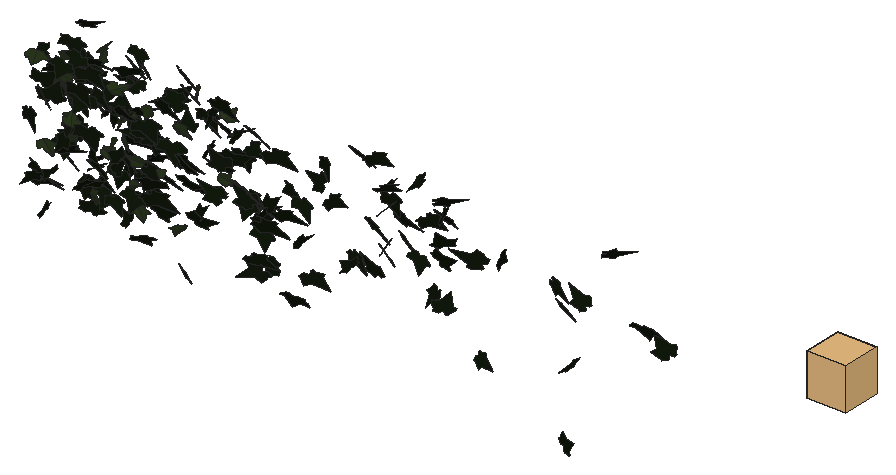
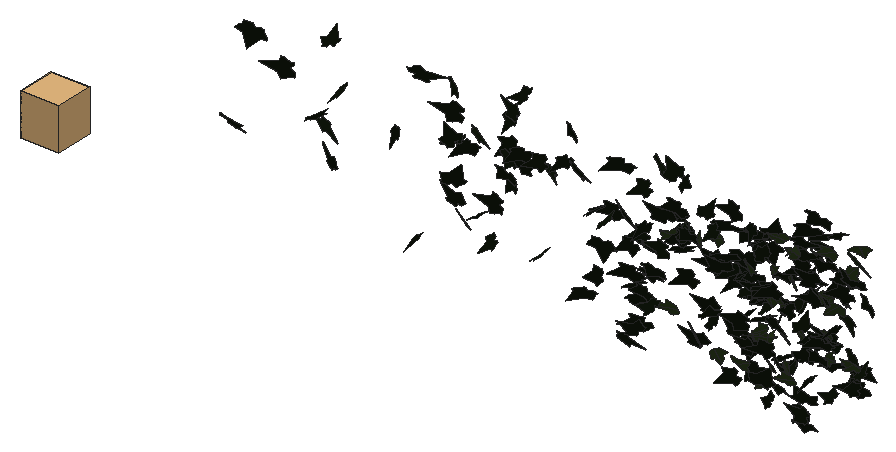
# SketchUp Ruby script. Lengths in millimetres.
U = 1.mm
M = Sketchup.active_model
def pt(a) = Geom::Point3d.new(a.map { |v| v * U })
def face(e, loops, mat)
  f = e.add_face(loops[0].map { |a| pt(a) })
  loops[1..].each { |l| e.add_face(l.map { |a| pt(a) }).erase! }
  f.material = f.back_material = mat if mat
  f
end
# faces: each face lists its corners as indices into pts; further lists are holes
def faces(e, pts, list, mat = nil) = list.each { |f| face(e, (f[0].is_a?(Array) ? f : [f]).map { |l| l.map { |i| pts[i] } }, mat) }
# xy, xz, yz: faces in a plane at the given z, y or x. An outline is a flat list of corners, or four numbers for a rectangle; further outlines are holes
def ring(l) = l.size == 4 ? [[l[0], l[1]], [l[2], l[1]], [l[2], l[3]], [l[0], l[3]]] : l.each_slice(2).to_a
def flat(e, list, mat, &to3) = list.each { |f| face(e, (f[0].is_a?(Array) ? f : [f]).map { |l| ring(l).map { |u, v| to3.(u, v) } }, mat) }
def xy(e, z, list, mat = nil) = flat(e, list, mat) { |x, y| [x, y, z] }
def xz(e, y, list, mat = nil) = flat(e, list, mat) { |x, z| [x, y, z] }
def yz(e, x, list, mat = nil) = flat(e, list, mat) { |y, z| [x, y, z] }
def lines(e, pts, list) = list.each { |a, b| e.add_line(pt(pts[a]), pt(pts[b])) }
# prism: a flat outline (further loops are holes) pulled along v
def prism(e, loops, v, mat = nil)
  f = face(e, loops, mat); d = Geom::Vector3d.new(v.map { |x| x * U })
  f.pushpull(f.normal.samedirection?(d) ? d.length : -d.length)
end
def box(e, o, s, mat = nil) = prism(e, [[o, [o[0] + s[0], o[1], o[2]], [o[0] + s[0], o[1] + s[1], o[2]], [o[0], o[1] + s[1], o[2]]]], [0, 0, s[2]], mat)
def at(x, y, z, deg = 0) = Geom::Transformation.translation(pt([x, y, z])) * Geom::Transformation.rotation(ORIGIN, Z_AXIS, deg.degrees)
def axes(o, x, y, z) = Geom::Transformation.new([*x, 0, *y, 0, *z, 0, *pt(o).to_a, 1])
def part(name) = M.definitions.add(name)
# library, detail: a bought-in or finely detailed component or shape, given as its bounding box
def library(name, o, s) = part(name).tap { |d| box(d.entities, o, s) }
def detail(e, o, s) = box(e.add_group.entities, o, s)
def put(e, d, t, mat = nil) = e.add_instance(d, t).tap { |i| i.material = mat if mat }
def group(e, t, mat = nil) = e.add_group.tap { |g| g.transformation = t; g.material = mat if mat }.entities
root = M.entities
M.materials.add("efeu1").color = [18, 25, 13]
M.materials.add("efeu2").color = [43, 57, 29]
c1 = part("ivyleaf_10")
p = [[0,12.8,-0.8],[-1.5,51.3,-10.9],[-4.9,51,-11.6],[-13.6,26.5,-7.3],[-13.2,15.9,-4.6],[-21.1,19.3,-7.2],
  [-29.5,16.3,-8.3],[-29.2,8.3,-6.2],[-19.7,-9.8,0.5],[-7.6,-13,4],[1,-12.2,5.8],[-0.4,51.1,-11.1],
  [-1.5,51.1,-10.9],[1,-12.4,5.9],[16.9,-12.4,3.5],[35.1,9.1,-5.1],[35,12.9,-6.1],[20.5,16.4,-4.9],
  [15.8,15,-3.8],[15.3,27.6,-7.1],[12.8,31.3,-7.8]]
faces(c1.entities,p,[[0,1,2,3,4,5,6,7,8,9,10],[11,12,0,13,14,15,16,17,18,19,20]],"efeu2")
c2 = part("ivyleaf_9")
p = [[39.1,54.8,31.7],[34.5,51.8,30.2],[-5.3,25.2,17.3],[-17.9,28.3,20.9],[-21.6,21.7,17],[-20.2,4.3,5.3],
  [-22.9,-0.3,2.5],[-17.1,-4,-0.6],[-2,-2.1,-1.2],[-0.7,-15.4,-10.1],[16.6,-22.3,-16.7],[21.1,-15.1,-12.5],
  [32.7,-10.7,-11],[46.1,-1.8,-6.6],[30.8,11.2,3.8]]
faces(c2.entities,p,[[0,1,2,3,4,5,6,7,8,9,10,11,12,13,14]],"efeu1")
c3 = library("Spot Light\#5",[-129.6,-129.6,-280.7],[259.2,259.2,280.7])
put(root,c1,axes([6203.9,621.5,2489.7],[-1.67739,0.69312,-0.54075],[-0.80083,0.3397,1.12123],[1.469,0.97662,-0.00622]))
put(root,c2,axes([6183.2,768,2235.6],[0.7316,-0.55002,-1.00228],[-0.6349,0.95744,-0.65335],[2.0812,0.48543,0.15301]))
put(root,c2,axes([6240.9,564.4,2556.4],[-1.99544,0.98431,-0.03793],[0.04978,-0.02755,-1.4381],[-1.87407,-1.04879,0.00218]))
put(root,c2,axes([6205.4,558.3,1839.3],[1.33312,-1.19278,-0.39127],[0.40774,-0.32789,1.38313],[-2.35406,-0.73227,0.01799]))
put(root,c1,axes([6179.7,635.3,1954.5],[1.88876,0.15588,0.66927],[1.25403,0.11796,-1.00451],[-0.37135,1.19117,0.0119]))
put(root,c1,axes([6211.5,798.8,2058],[0.12256,-0.72297,0.95503],[0.31658,-0.94174,-0.72413],[2.2576,0.17131,0.0497]))
put(root,c2,axes([6187.1,668.8,2400.7],[0.23122,0.78523,-1.06368],[0.17919,1.06031,0.7935],[2.50987,-0.14804,0.04134]))
put(root,c2,axes([6232.4,501.2,1847.8],[-0.12589,0.49094,-1.10293],[0.11335,-1.10191,-0.49406],[-2.29485,-0.08136,0.0361]))
put(root,c2,axes([6177.3,557.2,1786.8],[0.45038,0.37007,-1.21995],[1.32361,1.00242,0.43899],[2.03345,-0.73446,-0.01554]))
put(root,c2,axes([6189.4,791.5,1824],[0.92608,-0.93384,0.64277],[0.5601,-0.57145,-1.05301],[2.08364,0.56866,-0.00263]))
put(root,c2,axes([6200.5,891.4,2115.4],[-0.97149,-0.18358,-1.04783],[1.90164,0.31614,-0.54214],[0.69485,-1.12186,0.01869]))
put(root,c1,axes([6237.5,493.3,2574.2],[1.86344,0.72115,-0.31787],[-0.48416,-0.1906,-1.21602],[-1.41962,1.01162,-0.00252]))
put(root,c2,axes([6193.6,589.1,1783.7],[1.65973,-0.52992,0.60038],[1.00399,-0.28767,-1.02017],[1.14665,1.01893,0.02422]))
put(root,c1,axes([6224.6,709.8,2319.2],[-1.77312,-0.32143,-0.71865],[1.30965,0.2084,-0.98529],[0.72784,-1.15802,0.02216]))
put(root,c2,axes([6215.4,459.9,2237.4],[-0.9423,0.02108,-1.37483],[2.5765,-0.24824,-0.49134],[-0.45795,-1.44002,0.06457]))
put(root,c2,axes([6230.9,547.6,2381.5],[-1.24843,0.41545,1.05394],[1.69609,-0.56266,0.77646],[1.33113,1.10657,-0.00088]))
put(root,c2,axes([6218.1,907.7,2563.9],[1.53898,0.78591,-0.32463],[0.41404,0.24186,1.12743],[1.56447,-0.83712,0.02097]))
put(root,c2,axes([6270.2,706.9,1960.9],[-1.35456,-1.02965,-0.22299],[0.25219,0.17947,-1.25168],[1.98914,-0.72393,0.00685]))
put(root,c2,axes([6284,605.7,2330.6],[-1.67117,0.55744,-0.80683],[1.25082,-0.4693,-1.0395],[-1.38527,-1.09625,0.03474]))
put(root,c1,axes([6292.1,739.6,2361.1],[-0.49354,-0.31325,-1.17019],[-1.0474,-1.03561,0.39918],[-2.05387,0.6034,0.07762]))
put(root,c2,axes([6263.1,933.3,1750.8],[0.91761,1.1165,-0.16894],[0.05862,0.17062,1.21553],[2.1483,-0.48155,0.03899]))
put(root,c2,axes([6295.2,727.9,2572.3],[-1.47075,-0.62348,-0.78307],[1.0971,0.53156,-0.9921],[1.55741,-0.96324,-0.04062]))
put(root,c2,axes([6327.5,470.7,2318.5],[0.48347,-0.96814,0.77944],[-0.09839,0.78663,0.99392],[-2.36345,-0.23079,0.11807]))
put(root,c2,axes([6312.6,884.3,1743.7],[0.9635,0.90453,0.56899],[0.4437,0.52096,-1.0356],[-1.98479,0.55556,0.04471]))
put(root,c2,axes([6315.7,878.4,1669.7],[-1.75372,-0.42365,-0.59746],[1.03166,0.25125,-1.01418],[0.93742,-1.06907,-0.00159]))
put(root,c2,axes([6304,736.5,2347.7],[-0.97603,0.714,0.85246],[0.94774,-0.69189,0.87909],[1.89223,0.71482,-0.00059]))
put(root,c2,axes([6328.9,502.5,2333.5],[-1.9215,0.02098,0.93039],[1.75896,-0.13827,1.00603],[0.20756,1.36595,0.08755]))
put(root,c2,axes([6365.8,654.4,2044.4],[-2.15674,-0.05731,0.31312],[0.59618,0.00496,1.13462],[-0.10765,1.17567,0.01048]))
put(root,c2,axes([6317.9,707.2,2076],[-0.14127,-0.43959,-1.14988],[1.26939,0.95388,-0.40772],[1.96925,-0.64641,0.18033]))
put(root,c2,axes([6315.2,742.3,2347.8],[1.68353,-0.1317,0.83067],[1.56966,-0.1003,-0.89418],[0.31354,1.20931,0.0163]))
put(root,c2,axes([6377.4,725,2438.1],[-2.301,0.19968,0.29566],[0.55153,-0.0597,1.22534],[0.39606,1.24321,0.01135]))
put(root,c2,axes([6392,682.5,2124.8],[-2.29803,0.29739,-0.32961],[0.61206,-0.07253,-1.24352],[-0.58246,-1.24953,-0.00626]))
put(root,c1,axes([6374,622.8,2072.8],[-0.53915,-0.99616,-0.6593],[0.56517,0.59759,-1.03051],[2.20214,-0.39726,0.10306]))
put(root,c1,axes([6348.8,602.9,2562.1],[-1.38102,0.15262,-0.89165],[1.66715,-0.16683,-0.74143],[-0.42982,-1.13743,-0.0109]))
put(root,c2,axes([6354.2,564.7,2005.5],[1.77609,0.66225,0.92681],[1.32579,0.61617,-1.14171],[-1.71529,1.16198,0.07721]))
put(root,c2,axes([6393.5,750.4,2447.9],[-0.28012,0.10415,1.38679],[-1.38775,-1.19326,0.01223],[2.25379,-0.72179,0.17989]))
put(root,c2,axes([6373.9,815.9,2188.7],[1.73378,-1.00075,-0.24613],[0.31793,-0.18077,1.35328],[-1.93544,-0.92617,0.00182]))
put(root,c1,axes([6404.5,839.8,2448.7],[1.45414,-0.98172,0.0503],[-0.05538,0.04109,1.244],[-1.87004,-0.7646,0.00227]))
put(root,c2,axes([6452.4,609.7,2523.5],[-1.83124,0.81642,0.17396],[-0.26199,0.10664,-1.26186],[-1.56694,-0.97196,0.00768]))
put(root,c2,axes([6442.8,307.7,1782.9],[-0.99323,0.51634,-1.11801],[-1.48105,0.80283,0.73403],[1.81651,0.93689,-0.01283]))
put(root,c2,axes([6431.8,484,2581.6],[-1.29136,-1.07607,0.20661],[-0.20891,-0.17504,-1.27213],[2.0749,-0.68734,0.0005]))
put(root,c1,axes([6448.2,593.3,2289.1],[-0.09756,0.89413,-0.80109],[-0.30309,0.78966,0.89157],[2.2646,0.14421,0.08481]))
put(root,c1,axes([6433.9,542,2203.4],[1.08935,0.98736,-0.39768],[0.37086,0.34671,1.14125],[1.9916,-0.60462,0.005]))
put(root,c2,axes([6466.3,323.9,2005.8],[-0.37956,1.20599,0.54151],[-0.20139,0.53131,-1.22226],[-2.50793,-0.22518,0.01619]))
put(root,c2,axes([6408.6,719.5,2491.2],[2.09944,0.22395,0.4935],[0.91292,0.11736,-1.12547],[-0.47999,1.20275,0.01793]))
put(root,c1,axes([6414.4,863.1,1886],[0.61232,0.17186,1.13073],[2.00827,0.40847,-0.36233],[-0.8396,1.10237,-0.04203]))
put(root,c2,axes([6469.4,570.1,2597],[-1.40195,-0.95933,0.42304],[-0.4398,-0.35574,-1.20911],[1.94637,-0.77138,0.0315]))
put(root,c2,axes([6454.5,637.4,1782.8],[0.83229,-0.7398,-1.03712],[-0.86945,0.93253,-0.85782],[2.26331,0.63028,0.05185]))
put(root,c1,axes([6471.6,743.1,2566.4],[0.2876,-0.9727,0.69265],[0.23928,0.70725,0.96577],[-2.26,-0.0489,0.1904]))
put(root,c2,axes([6457.9,466.6,2433],[0.74451,-0.26758,-1.36632],[2.33775,-0.60184,0.46954],[-1.2475,-1.2875,0.06448]))
put(root,c2,axes([6480.2,654.6,1646.6],[-1.47719,-0.0401,1.00768],[1.89375,-0.23741,0.75697],[0.31239,1.24959,0.17616]))
put(root,c2,axes([6495.7,930.4,1758.7],[-0.15346,-0.10995,1.24239],[1.31677,1.03194,0.13623],[-1.97507,0.69653,-0.00571]))
put(root,c2,axes([6550.7,854.2,2195.7],[-0.24041,0.01454,-1.19902],[-2.28163,-0.02682,0.12597],[-0.04787,1.20535,0.01727]))
put(root,c1,axes([6519.8,771.9,1895],[0.64652,-1.19723,0.22203],[0.12271,-0.2125,-1.24448],[2.31416,0.34574,0.00396]))
put(root,c2,axes([6513.1,383.8,2210.2],[0.27489,-0.16201,-1.36442],[1.30272,-1.18109,0.2127],[-2.2674,-0.69823,-0.04321]))
put(root,c2,axes([6513.7,724.9,2204.8],[0.50272,0.18887,1.19966],[1.23897,1.0144,-0.30304],[-1.95119,0.69279,0.11666]))
put(root,c2,axes([6524.9,841.3,1809.7],[-1.78641,-0.0812,-0.74508],[1.41067,0.07648,-0.94209],[0.2115,-1.19597,-0.00965]))
put(root,c2,axes([6529,585.5,1845.5],[1.69103,0.37828,0.81149],[-1.42084,-0.31809,0.96569],[0.94064,-1.16052,-0.00018]))
put(root,c2,axes([6530.5,681.5,1844.4],[1.57513,-0.64744,-0.86758],[-1.20735,0.59484,-1.04907],[1.66944,1.04106,0.05987]))
put(root,c2,axes([6594.7,578,2525.4],[-0.94832,0.04659,1.06697],[-2.02693,0.06613,-0.50025],[-0.15159,-1.17572,0.01414]))
put(root,c2,axes([6559.3,922.2,1845],[1.77725,-0.21529,0.81178],[-1.50403,0.18568,0.95831],[-0.54105,-1.22333,0.00259]))
put(root,c2,axes([6557,732.1,2207.1],[0.80979,-0.30275,-1.14645],[-1.56115,0.8044,-0.51686],[1.6296,0.92105,0.07455]))
put(root,c2,axes([6528.7,850.8,2378.9],[2.31642,0.15965,0.26245],[0.49545,0.03331,-1.22755],[-0.3104,1.24465,-0.00081]))
put(root,c2,axes([6552.5,466.8,1905.7],[-0.17538,0.79079,-1.01641],[-0.37201,0.99861,0.79466],[2.42254,0.2106,0.04845]))
put(root,c2,axes([6552.2,764.6,1858.8],[-0.67605,0.88898,0.8258],[0.3177,-0.81648,0.95075],[2.28731,0.37616,0.11202]))
put(root,c2,axes([6568,714.3,2395.5],[-1.6415,-0.80279,-0.27239],[0.37685,0.18706,-1.17829],[1.56881,-0.88493,-0.00197]))
put(root,c2,axes([6565.8,501,2582.8],[-0.59664,-0.55199,-1.21016],[1.12797,1.05511,-0.63479],[2.26627,-0.67047,-0.00265]))
put(root,c2,axes([6607.5,448.4,2460.2],[-2.28289,-0.83443,-0.04972],[0.09398,0.01608,-1.46111],[1.58813,-1.20042,0.01499]))
put(root,c2,axes([6557.2,858.6,2012.3],[1.82213,-0.11575,0.72856],[1.39177,-0.00818,-0.96228],[0.18478,1.20306,0.06355]))
put(root,c1,axes([6625,766.6,2025.8],[-0.24829,0.74801,-1.01828],[-0.6983,0.95715,0.75012],[2.30106,0.37118,0.11776]))
put(root,c2,axes([6622.5,735.4,2248.9],[-2.47065,0.31772,0.36336],[0.66894,-0.09235,1.33646],[0.62962,1.34489,0.00593]))
put(root,c2,axes([6637,851.9,2346.3],[-1.67537,-0.80384,0.22475],[0.32836,0.14435,1.19204],[-1.55423,0.89699,0.00957]))
put(root,c2,axes([6611.9,515.9,2086.6],[-0.35427,-0.2685,1.46453],[-0.60116,-1.43522,-0.30327],[2.76925,-0.34591,0.12152]))
put(root,c1,axes([6612.6,830.5,2107.4],[0.13336,0.14711,1.19445],[0.15472,1.19316,-0.15172],[-2.28522,0.08937,0.05943]))
put(root,c2,axes([6659.8,659.2,2020.7],[-0.70392,0.93071,0.81343],[-0.6045,0.74899,-1.0014],[-2.2735,-0.48731,0.01441]))
put(root,c2,axes([6629.3,622.3,1807],[-1.24839,-1.11147,0.48067],[-0.42418,-0.42651,-1.29038],[2.26531,-0.69239,0.02327]))
put(root,c1,axes([6623.7,807.8,1780],[-0.3492,-0.43758,-1.10288],[0.83329,1.01226,-0.47446],[2.09881,-0.4747,0.00488]))
put(root,c1,axes([6629.2,749.2,2259.4],[2.40019,-0.01434,0.0856],[0.16308,0.00762,-1.26119],[0.02624,1.26401,0.00857]))
put(root,c2,axes([6614.4,515.6,2461.9],[1.15963,-1.12139,-0.48044],[-0.29437,0.46169,-1.27378],[2.30312,0.62363,0.0791]))
put(root,c2,axes([6618.5,360.6,2567.8],[-1.1476,-0.24379,-1.24831],[2.18454,0.49083,-0.6503],[1.0428,-1.29652,-0.01146]))
put(root,c1,axes([6653.6,627.6,2124.7],[0.24898,-0.25494,1.16798],[0.76443,-1.09728,-0.2845],[2.14297,0.42104,-0.03422]))
put(root,c2,axes([6680.8,713.4,2538.2],[1.02708,1.06788,-0.68334],[-0.62904,-0.59849,-1.19629],[-2.32944,0.63246,0.02175]))
put(root,c2,axes([6662,772.3,2246.6],[-0.65415,-1.10084,0.46067],[-0.21504,-0.44722,-1.15301],[2.26096,-0.36104,0.02362]))
put(root,c1,axes([6648,462.7,1881.6],[-0.04848,0.04758,-1.24777],[1.07905,-1.11152,-0.05396],[-2.11739,-0.56754,0.00107]))
put(root,c1,axes([6729.7,737.7,1985.3],[-0.73072,-0.04178,-1.20552],[-2.2842,-0.11329,0.38617],[-0.2296,1.2601,-0.00525]))
put(root,c2,axes([6647.5,793.9,2515.1],[0.57356,-0.78689,1.13604],[0.75279,-1.06499,-0.8426],[2.5201,0.49721,-0.00686]))
put(root,c2,axes([6672.8,808.7,2602.5],[-0.34955,-1.20134,0.11107],[-0.01162,-0.11142,-1.21525],[2.29612,-0.18345,0.01076]))
put(root,c2,axes([6689.1,467.1,2049.6],[1.32195,-1.25849,-0.18746],[0.24894,-0.14182,1.43673],[-2.40876,-0.70533,0.0456]))
put(root,c2,axes([6678.9,590.3,1814.9],[-0.09919,-1.08216,-0.44479],[0.03347,0.44446,-1.08341],[2.22651,-0.05489,-0.00353]))
put(root,c2,axes([6687.9,362.2,2328.2],[-1.39169,-0.71709,-0.95676],[1.25345,0.69446,-1.02385],[1.89924,-0.98378,-0.02536]))
put(root,c1,axes([6749.7,866.9,1864.7],[1.79409,-0.03003,0.77871],[-1.4749,0.09259,0.9417],[-0.1562,-1.2192,0.05234]))
put(root,c2,axes([6692.5,749.1,2271.5],[0.99154,0.99348,-0.59587],[0.4364,0.55199,1.12081],[2.16119,-0.56726,0.04706]))
put(root,c1,axes([6739.5,595.8,2316],[0.3376,-1.1205,0.34459],[0.13246,-0.33783,-1.13435],[2.22716,0.18994,0.01523]))
put(root,c2,axes([6754.8,705.5,2502.8],[-0.94132,0.95537,-0.5898],[0.52752,-0.52065,-1.07579],[-2.07071,-0.56694,-0.00594]))
put(root,c2,axes([6776.5,712.9,2175.9],[-0.92701,-0.13914,1.16323],[-2.089,-0.38615,-0.5058],[0.77938,-1.20052,0.02787]))
put(root,c1,axes([6706.3,556.9,2494.8],[0.83586,0.28464,-1.10778],[1.80529,0.57241,0.52314],[1.21633,-1.04519,-0.01518]))
put(root,c2,axes([6734.1,922.2,1825.7],[2.38289,-0.20932,0.08423],[0.16148,-0.00328,-1.26937],[0.3979,1.25487,0.01073]))
put(root,c2,axes([6800.8,567.1,1736],[-1.2203,0.35245,-0.99221],[-1.64578,0.48655,0.73165],[1.14338,1.0765,-0.00583]))
put(root,c2,axes([6793.8,700.5,2594.3],[1.48114,-0.30414,-0.90228],[-1.61046,0.31337,-0.83549],[0.83086,1.14959,-0.01096]))
put(root,c2,axes([6793,594.7,2052.7],[-0.1921,-0.80205,1.017],[0.0152,-1.02045,-0.80398],[2.46501,-0.05621,0.08421]))
put(root,c2,axes([6833.7,647.8,1870.9],[1.65725,0.943,-0.26104],[-0.33432,-0.1931,-1.28355],[-1.83196,0.88831,-0.00191]))
put(root,c1,axes([6830.5,693.1,2358.3],[1.71777,-0.82679,0.12869],[0.18649,-0.08355,-1.224],[1.58153,0.90786,0.00455]))
put(root,c2,axes([6791.5,728,1885],[1.28507,-0.24603,-1.04616],[2.03794,0.0488,0.67964],[-0.17419,-1.24418,0.23353]))
put(root,c2,axes([6833.9,472,2421],[2.17714,-0.56801,0.34023],[-0.56954,0.16232,1.27714],[-1.12409,-1.18237,0.01188]))
put(root,c2,axes([6817.9,745.1,2042.2],[0.9293,0.94128,-0.71449],[0.62404,0.63481,1.06039],[2.16078,-0.58816,0.00104]))
put(root,c2,axes([6860.8,680.7,2162.8],[1.14777,-1.12311,-0.10996],[0.15757,-0.08031,1.27431],[-2.14194,-0.60774,0.03482]))
put(root,c2,axes([6843.7,621.8,2227.3],[-1.04775,0.13223,1.13004],[2.00652,-0.41265,0.5619],[0.81403,1.18734,0.06943]))
put(root,c2,axes([6886.4,955.9,2148.5],[-1.44087,-0.64526,0.84904],[1.25119,0.53746,0.99466],[-1.59806,1.00259,0.01323]))
put(root,c2,axes([6865.9,645.9,2037.1],[0.82945,-0.97376,-0.90291],[-0.70382,0.8237,-1.06683],[2.42737,0.57157,-0.0008]))
put(root,c2,axes([6878.3,558.3,1665.5],[1.82017,0.78651,0.07735],[0.11299,0.04958,-1.23825],[-1.49986,0.95821,0.00058]))
put(root,c2,axes([6889.9,513.4,1939.3],[-1.12677,-1.25495,0.25151],[-0.15368,-0.23993,-1.38729],[2.43107,-0.59683,0.02887]))
put(root,c1,axes([6872.5,557.4,1834.7],[2.15506,-0.03499,0.50113],[0.95401,-0.00262,-1.13281],[0.06291,1.23827,0.01177]))
put(root,c2,axes([6923.9,650.3,2234.1],[-0.89926,-0.58932,1.07726],[-1.20064,-0.87378,-0.75471],[2.00498,-0.78756,0.03122]))
put(root,c2,axes([6887.1,847.1,2377.6],[-0.94965,-0.18742,1.24288],[2.33061,0.22896,0.52615],[-0.53925,1.31958,0.08523]))
put(root,c2,axes([6886.2,534.5,2064.3],[0.80319,-0.97905,0.86332],[0.62036,-0.79954,-1.06605],[2.40559,0.53308,-0.01333]))
put(root,c2,axes([6940,640.4,2211.9],[0.3075,-0.24738,-1.42447],[-0.81007,1.36167,-0.28475],[2.62968,0.44839,0.07885]))
put(root,c2,axes([6935.8,509.9,2077.3],[0.37412,-1.35624,0.37835],[0.18459,-0.36807,-1.36978],[2.67339,0.21521,0.04163]))
put(root,c2,axes([6951.4,815.1,2572.2],[2.02404,-0.69891,-0.48286],[-0.77074,0.26298,-1.27259],[1.42121,1.13798,-0.00247]))
put(root,c2,axes([6940.3,640,2253.5],[2.4141,-0.32266,0.13001],[0.24282,-0.0258,-1.30882],[0.61592,1.27483,0.00642]))
put(root,c2,axes([6970.4,488.6,2415.6],[-1.0207,-0.87006,-1.01848],[0.93149,0.89395,-1.02139],[2.3731,-0.72512,-0.03715]))
put(root,c2,axes([7068.5,660.9,2499.4],[-1.92478,-0.30167,1.02001],[-1.87364,-0.26753,-1.05522],[0.76662,-1.41126,-0.018]))
put(root,c2,axes([6979.9,582.5,1844.3],[-0.11123,-0.09754,1.41171],[1.68607,-1.10428,-0.03962],[2.10008,0.88142,0.10658]))
put(root,c1,axes([7063.1,672.9,1742.1],[-0.84308,-1.11351,0.31678],[-0.2344,-0.29193,-1.19837],[2.19082,-0.45974,-0.00631]))
put(root,c1,axes([7050.2,831.1,2492.2],[0.37206,-0.31815,1.19268],[1.17905,-1.01917,-0.37341],[2.03199,0.64962,-0.00171]))
put(root,c2,axes([7035.9,533.8,2537.3],[0.46605,0.03114,-1.3683],[2.59052,0.13996,0.24678],[0.27265,-1.38298,-0.00584]))
put(root,c2,axes([7074.9,585.3,2279.6],[-1.13673,-1.18153,-0.5536],[0.41664,0.50947,-1.32353],[2.44807,-0.63533,-0.0318]))
put(root,c2,axes([7117,365.9,2169.9],[1.34797,1.03381,-0.84738],[-1.0109,-0.66236,-1.25205],[-2.33458,0.88373,0.05288]))
put(root,c2,axes([7074.4,688.9,2008],[0.60227,-0.33114,1.15761],[1.77466,-0.68983,-0.45223],[1.44974,0.98201,0.07268]))
put(root,c2,axes([7128.7,682.4,2547.8],[1.31974,-1.07414,0.27797],[-0.27233,0.23848,1.2785],[-2.09402,-0.70798,0.00892]))
put(root,c1,axes([7098.2,604.2,2383.5],[-0.93089,0.33884,-1.09093],[1.78472,-0.5586,-0.59394],[-1.24156,-1.05704,-0.03583]))
put(root,c2,axes([7107.7,379.1,2074.3],[-0.06357,-0.29208,-1.48571],[1.49942,1.26571,-0.26654],[2.46091,-0.77874,0.12402]))
put(root,c2,axes([7131.7,733.9,1810.3],[-0.15421,0.94529,0.90342],[0.09421,-0.90228,0.94854],[2.48678,0.0928,0.02009]))
put(root,c2,axes([7102.1,585.6,2211.8],[0.75207,0.11839,-1.36777],[2.32804,0.61585,0.4067],[1.18631,-1.28362,0.06898]))
put(root,c2,axes([7134.7,709.8,1791.1],[0.14669,-0.07267,1.29043],[1.98323,-0.76125,-0.10511],[1.45518,1.04481,0.01317]))
put(root,c2,axes([7146,566.8,2205.5],[0.68207,-0.58247,1.2473],[1.1094,-1.10341,-0.68276],[2.37347,0.68314,-0.0393]))
put(root,c2,axes([7183.1,740.6,2439.3],[-1.16394,-0.25419,-1.10463],[1.95133,0.41114,-0.66226],[0.91985,-1.19381,0.00713]))
put(root,c2,axes([7223.3,718.8,2387.1],[1.79698,-0.67248,-0.66365],[1.02382,-0.38867,1.15919],[-1.47824,-1.08668,-0.00391]))
put(root,c1,axes([7217.2,835,2019],[0.65802,0.02935,1.20866],[2.21242,0.33738,-0.34073],[-0.63231,1.21102,0.06563]))
put(root,c1,axes([7274.9,788.5,2424.6],[0.95766,0.5879,-0.99875],[1.02232,0.8465,0.7689],[1.95445,-0.73084,0.08718]))
put(root,c2,axes([7282,597.7,2077.5],[1.69402,0.57239,0.75218],[1.20097,0.40938,-1.05825],[-1.33931,1.09108,0.00245]))
put(root,c2,axes([7329.2,569.2,2348.1],[-0.37862,0.28865,-1.40935],[-1.63927,1.11567,0.35008],[2.19299,0.88381,0.01837]))
put(root,c2,axes([7276.3,711.4,2551.9],[-0.16939,-0.06093,-1.33903],[2.37377,0.4878,-0.1051],[0.93446,-1.25019,0.02425]))
put(root,c2,axes([7308,798.5,2326.1],[0.34276,1.12591,-0.5523],[0.08641,0.55174,1.13959],[2.38519,-0.18178,0.03808]))
put(root,c2,axes([7313.3,383.5,1694.6],[1.39142,-0.66925,-0.85109],[1.41217,-0.43817,0.98194],[-1.50062,-1.03289,0.1349]))
put(root,c2,axes([7349.8,834.1,2214.7],[-1.42688,-0.31351,-0.98532],[1.71736,0.39589,-0.81256],[0.96087,-1.17312,-0.01089]))
put(root,c2,axes([7378.1,550.9,2600.6],[-0.33251,0.28734,-1.27841],[1.48819,-1.01203,-0.33433],[-2.00103,-0.8004,-0.03621]))
put(root,c2,axes([7344.8,848,1989.6],[1.31457,-1.13036,0.40509],[0.45569,-0.32829,-1.32431],[2.23938,0.73035,0.03168]))
put(root,c2,axes([7388.5,593.2,2253.1],[2.19431,-0.35702,0.50322],[-0.8879,0.1935,1.2062],[-0.76847,-1.24302,0.04324]))
put(root,c2,axes([7461.4,496.6,2138.3],[-1.70083,-1.02299,-0.11982],[-0.15061,-0.08998,1.35836],[-1.95446,0.89717,-0.0004]))
put(root,c2,axes([7491.2,500.3,2337.3],[-2.33903,-0.12499,-0.3778],[-0.71577,-0.03593,1.23534],[-0.24748,1.28525,-0.0022]))
put(root,c2,axes([7437.5,866.2,1825.2],[-0.10865,-0.07814,1.27897],[2.23978,0.50322,0.08328],[-0.96465,1.1772,0.0493]))
put(root,c2,axes([7439.7,785.2,2022.1],[-0.13887,-0.1971,-1.26169],[2.37511,0.25693,-0.11231],[0.51528,-1.2374,0.17765]))
put(root,c2,axes([7475.7,489.8,2578.6],[2.2611,-0.46251,-0.71038],[1.2627,-0.25392,1.2749],[-1.00415,-1.36075,0.00356]))
put(root,c2,axes([7507.7,705.5,2362.7],[0.4602,-0.56988,-1.33838],[-0.94988,1.24189,-0.61896],[2.60045,0.55448,0.01076]))
put(root,c2,axes([7528.1,658.6,2054.8],[-2.07786,-0.34123,-0.57667],[1.06404,0.1438,-1.14355],[0.70295,-1.22631,0.02637]))
put(root,c2,axes([7489.1,561,2346.5],[-0.36904,0.01017,1.3096],[2.30797,-0.49851,0.18343],[0.94119,1.22643,0.0637]))
put(root,c2,axes([7622.5,560.9,2134.3],[-2.38927,-0.07984,-0.57226],[-1.08756,-0.03104,1.25792],[-0.16277,1.37932,-0.00482]))
put(root,c2,axes([7635.3,748.3,1672.5],[-1.20291,-0.11207,-1.16735],[-2.15409,-0.28881,0.64054],[-0.58421,1.29567,0.04181]))
put(root,c2,axes([7563.9,657.2,1743.6],[0.17028,-0.06594,-1.32036],[1.22489,1.15813,-0.01423],[2.19774,-0.64037,0.11023]))
put(root,c2,axes([7566.7,617.5,2527.7],[2.28464,-0.60886,0.02526],[0.04614,-0.00805,-1.34599],[1.15886,1.20066,0.00379]))
put(root,c2,axes([7622.1,433.9,2574.2],[0.04688,0.83925,1.01161],[0.04813,1.0113,-0.83961],[-2.50114,0.03519,0.00281]))
put(root,c2,axes([7646.6,636.1,1930.6],[-0.59615,-1.2984,-0.05208],[0.02617,0.05026,-1.33564],[2.47296,-0.31354,0.00158]))
put(root,c2,axes([7646.6,536.6,2187.7],[2.33535,-0.79712,0.04283],[0.06931,-0.02257,-1.46324],[1.51768,1.2276,0.00091]))
put(root,c2,axes([7725.9,515.6,1782.1],[-0.0779,-0.16407,-1.34851],[-0.59036,-1.31235,0.16909],[-2.5171,0.31287,0.00207]))
put(root,c2,axes([7655.2,619.9,1995.6],[-0.01342,0.00792,-1.38544],[1.72433,1.04818,0.00138],[1.99486,-0.90598,-0.01051]))
put(root,c2,axes([7713.4,561.4,2115.9],[-0.30747,0.6613,-1.1569],[-0.56862,1.11773,0.68063],[2.47158,0.33941,0.01267]))
put(root,c2,axes([7788,495.2,2197.4],[-0.49148,0.93084,0.99709],[0.50789,-0.96071,0.966],[2.54591,0.37135,-0.00023]))
put(root,c2,axes([7828.2,658,2236.6],[1.00693,-1.03457,-0.70881],[0.68406,-0.61195,1.16146],[-2.28666,-0.63864,0.03533]))
put(root,c2,axes([7844.8,666.5,1919.1],[0.49852,0.35802,1.28119],[1.5126,1.005,-0.44333],[-2.03025,0.83667,-0.01571]))
put(root,c2,axes([7826.5,492.4,2529.8],[-0.18795,-0.42717,-1.39353],[1.10069,1.27058,-0.43047],[2.54626,-0.58078,0.08322]))
put(root,c2,axes([7895.4,463,2211.4],[0.28996,0.2178,-1.29973],[1.52564,1.02318,0.26542],[1.99077,-0.81584,-0.0141]))
put(root,c2,axes([7944.7,581.7,2245],[0.12501,-1.40203,-0.1705],[-0.04389,0.16959,-1.40349],[2.68764,0.06798,-0.01499]))
put(root,c2,axes([7956.6,640.7,1780.3],[-0.06295,-0.55754,-1.23541],[0.50558,1.20914,-0.5528],[2.52955,-0.25554,0.07974]))
put(root,c2,axes([8110.1,548.3,2428.4],[-1.31612,0.17175,-1.23057],[-2.29372,0.24979,0.71213],[0.5751,1.38929,0.02409]))
put(root,c2,axes([8121,294.2,1861.9],[1.88116,0.49753,-0.81601],[-1.40523,-0.34785,-1.10645],[-1.15493,1.23363,0.01712]))
put(root,c2,axes([8142.8,771.8,2543.7],[2.23296,-0.61221,0.19114],[0.31462,-0.09636,-1.32336],[1.17939,1.18482,-0.00887]))
put(root,c2,axes([8168.7,492.7,2606.7],[-0.86071,0.10993,-1.24466],[2.29299,-0.31252,-0.46536],[-0.63038,-1.28687,0.00669]))
put(root,c2,axes([8187.9,714.8,1956],[0.97743,-1.27302,-0.3118],[-0.23778,0.28581,-1.37268],[2.48306,0.52848,-0.00871]))
put(root,c2,axes([8226.3,473.3,2403],[0.31634,-0.21391,-1.36498],[-0.71036,1.31675,-0.2518],[2.53176,0.39618,0.0999]))
put(root,c2,axes([8280.2,763.5,2551.8],[-0.05053,-0.17538,-1.33524],[0.06123,1.33503,-0.17599],[2.56232,-0.03536,-0.02213]))
put(root,c2,axes([8375.9,892.6,2045.7],[2.04811,-0.7505,-0.53072],[-0.82768,0.30419,-1.312],[1.54122,1.16069,0.00068]))
put(root,c2,axes([8419.9,701.4,2445.7],[0.4022,0.92172,0.96386],[0.33631,0.94793,-0.94523],[-2.51581,0.27407,0.02774]))
put(root,c2,axes([8414.6,737.4,2372.9],[-1.16643,-0.16285,-1.20292],[2.25878,0.20255,-0.6321],[0.48508,-1.33477,0.05084]))
put(root,c2,axes([8438.3,632,2479.3],[1.70112,0.83853,0.7263],[0.99741,0.50291,-1.22556],[-1.86086,1.03611,0.00707]))
put(root,c2,axes([8403.4,818,2221.6],[1.17504,0.11947,-1.3361],[2.53299,0.12929,0.62656],[0.31912,-1.46616,-0.05362]))
put(root,c2,axes([8512.5,278,2183.6],[-0.48753,1.26819,0.69926],[-0.40891,0.66898,-1.29197],[-2.72571,-0.32719,0.06875]))
put(root,c2,axes([8539.5,536.3,2195.9],[-0.68874,0.50533,-1.32946],[-1.57436,1.04113,0.62091],[2.2019,0.90248,0.0281]))
put(root,c2,axes([8630.1,348.6,2159.5],[0.45022,-0.37698,1.31168],[-1.33936,1.10692,0.44505],[-2.22551,-0.74243,-0.00248]))
put(root,c2,axes([8593.9,760.4,2062.9],[-0.51772,-1.31142,0.28322],[-0.12374,-0.27576,-1.33931],[2.55043,-0.27959,-0.00749]))
put(root,c2,axes([8628.2,735.3,2548.1],[-1.77798,0.83294,-0.57523],[0.72615,-0.43529,-1.24995],[-1.78445,-1.00705,0.06451]))
put(root,c2,axes([8627.3,397.1,2499.8],[0.60984,1.26118,0.47547],[-0.34385,-0.44412,1.29978],[2.54204,-0.36263,0.06175]))
put(root,c2,axes([8676.5,246.4,2529.4],[1.69624,-1.17957,0.11251],[0.14415,-0.08379,-1.47839],[2.25053,0.89442,0.00989]))
put(root,c2,axes([8729.9,651.2,2392.1],[-0.08981,-0.32931,-1.41762],[0.01044,1.41831,-0.32966],[2.76983,-0.01602,-0.04472]))
put(root,c2,axes([8765.8,748.7,2199.2],[1.44941,0.31198,1.10789],[-1.93813,-0.43645,0.82292],[1.02085,-1.27158,-0.01063]))
put(root,c2,axes([8773.4,672.2,1959.9],[-1.92548,0.44939,-0.82201],[1.38209,-0.38816,-1.10598],[-1.12644,-1.24442,0.04813]))
put(root,c2,axes([8758.3,254.8,2378.1],[2.12262,-0.51033,-0.84508],[-1.45573,0.3594,-1.22648],[1.18787,1.35236,0.00704]))
put(root,c2,axes([8735.7,750.9,2092.9],[-0.25246,0.11052,1.36883],[1.42237,-1.14791,0.16511],[2.1927,0.75736,0.0505]))
put(root,c2,axes([8800.4,691.3,2404.9],[2.32833,-0.35894,-0.52729],[0.97349,-0.12937,1.27481],[-0.72531,-1.32587,0.01836]))
put(root,c2,axes([8829.5,622.4,2535.4],[1.0867,1.13163,-0.73366],[0.55319,0.67472,1.26694],[2.50642,-0.63955,0.03846]))
put(root,c2,axes([8995.3,453.4,2575.9],[-0.8252,0.64062,-1.22328],[-1.78779,0.80295,0.75345],[1.9263,1.01965,0.17523]))
put(root,c2,axes([9098.6,626.7,1699.2],[0.92947,-0.75388,-1.08236],[-1.03421,0.93668,-0.8976],[2.28744,0.72982,0.03397]))
put(root,c2,axes([9110.7,310.3,2123.4],[-1.3539,-0.40007,1.16251],[1.87532,0.61767,0.81554],[-1.39929,1.21489,-0.03181]))
put(root,c2,axes([9213.9,661.9,2315],[0.16747,-0.12986,-1.44929],[-1.83292,1.08321,-0.15553],[2.07596,0.96687,-0.0204]))
put(root,c2,axes([9332.2,339.7,2469.1],[-0.79967,0.08164,1.37651],[-2.57644,0.24936,-0.42801],[-0.49931,-1.41744,0.00398]))
put(root,c2,axes([9647.8,564.5,2362.6],[1.54854,-1.04801,-0.70223],[-0.81436,0.55682,-1.32678],[2.25862,0.9193,0.00308]))
put(root,c2,axes([9749.5,692.8,2210.8],[-1.4574,-1.15652,0.4312],[0.45105,0.36023,1.38706],[-2.30539,0.8016,-0.00121]))
put(root,c2,axes([9893,424.9,2022.8],[-1.3518,1.21898,-0.38659],[0.37868,-0.33149,-1.41081],[-2.40421,-0.73761,-0.00485]))
put(root,c2,axes([9841.5,772.9,2514.7],[0.70414,1.09419,-0.91304],[0.52656,0.87021,1.15497],[2.66063,-0.4618,0.01306]))
put(root,c2,axes([9945.2,297,2421.2],[1.78616,-1.11849,-0.28538],[0.36963,-0.20956,1.46],[-2.16559,-0.95829,0.01382]))
put(root,c2,axes([9979,234.3,1646.6],[-0.12803,0.38205,1.42749],[0.48697,-1.40438,0.38792],[2.76994,0.26456,-0.00222]))
put(root,c2,axes([10249.1,771.3,2057],[-2.54801,0.25344,-0.64629],[-1.2041,0.13247,1.36253],[0.54384,1.48072,-0.01127]))
put(root,c2,axes([10357.4,415.2,2410.6],[2.47137,0.47011,-0.56943],[-1.02256,-0.18869,-1.381],[-0.96403,1.40529,0.00506]))
put(root,c3,at(11042.6,1226.8,2166.9))
